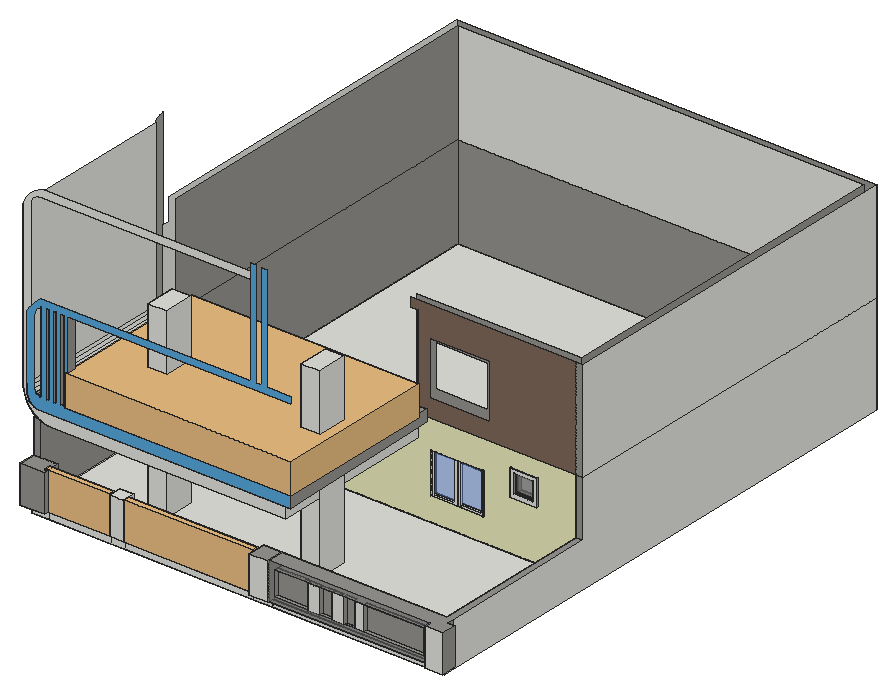
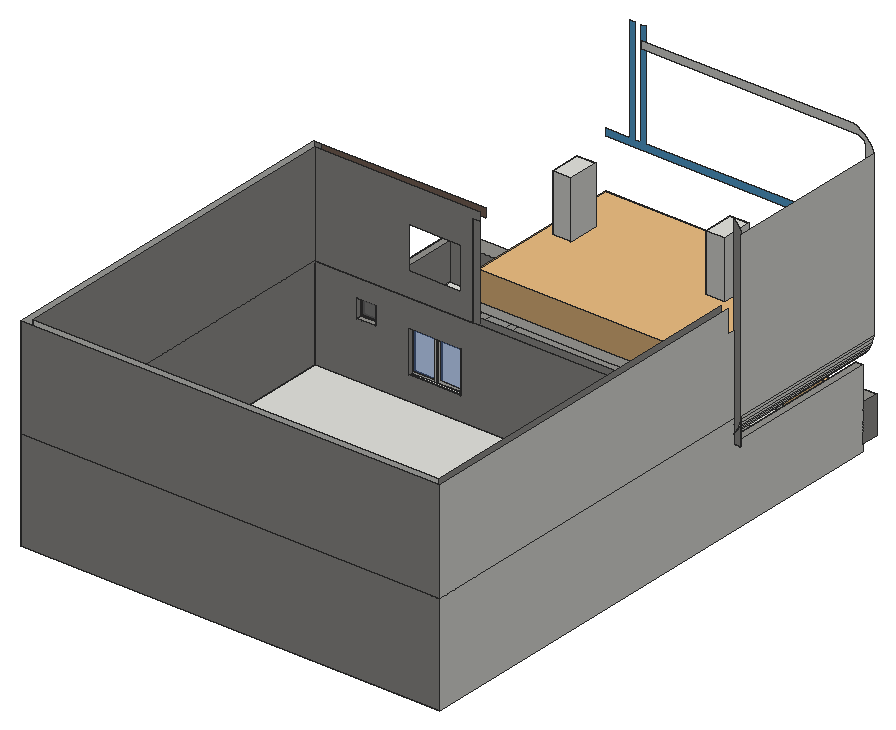
# SketchUp Ruby script. Lengths in millimetres.
U = 1.mm
M = Sketchup.active_model
def pt(a) = Geom::Point3d.new(a.map { |v| v * U })
def face(e, loops, mat)
  f = e.add_face(loops[0].map { |a| pt(a) })
  loops[1..].each { |l| e.add_face(l.map { |a| pt(a) }).erase! }
  f.material = f.back_material = mat if mat
  f
end
# faces: each face lists its corners as indices into pts; further lists are holes
def faces(e, pts, list, mat = nil) = list.each { |f| face(e, (f[0].is_a?(Array) ? f : [f]).map { |l| l.map { |i| pts[i] } }, mat) }
# xy, xz, yz: faces in a plane at the given z, y or x. An outline is a flat list of corners, or four numbers for a rectangle; further outlines are holes
def ring(l) = l.size == 4 ? [[l[0], l[1]], [l[2], l[1]], [l[2], l[3]], [l[0], l[3]]] : l.each_slice(2).to_a
def flat(e, list, mat, &to3) = list.each { |f| face(e, (f[0].is_a?(Array) ? f : [f]).map { |l| ring(l).map { |u, v| to3.(u, v) } }, mat) }
def xy(e, z, list, mat = nil) = flat(e, list, mat) { |x, y| [x, y, z] }
def xz(e, y, list, mat = nil) = flat(e, list, mat) { |x, z| [x, y, z] }
def yz(e, x, list, mat = nil) = flat(e, list, mat) { |y, z| [x, y, z] }
def lines(e, pts, list) = list.each { |a, b| e.add_line(pt(pts[a]), pt(pts[b])) }
# prism: a flat outline (further loops are holes) pulled along v
def prism(e, loops, v, mat = nil)
  f = face(e, loops, mat); d = Geom::Vector3d.new(v.map { |x| x * U })
  f.pushpull(f.normal.samedirection?(d) ? d.length : -d.length)
end
def box(e, o, s, mat = nil) = prism(e, [[o, [o[0] + s[0], o[1], o[2]], [o[0] + s[0], o[1] + s[1], o[2]], [o[0], o[1] + s[1], o[2]]]], [0, 0, s[2]], mat)
def at(x, y, z, deg = 0) = Geom::Transformation.translation(pt([x, y, z])) * Geom::Transformation.rotation(ORIGIN, Z_AXIS, deg.degrees)
def axes(o, x, y, z) = Geom::Transformation.new([*x, 0, *y, 0, *z, 0, *pt(o).to_a, 1])
def part(name) = M.definitions.add(name)
# library, detail: a bought-in or finely detailed component or shape, given as its bounding box
def library(name, o, s) = part(name).tap { |d| box(d.entities, o, s) }
def detail(e, o, s) = box(e.add_group.entities, o, s)
def put(e, d, t, mat = nil) = e.add_instance(d, t).tap { |i| i.material = mat if mat }
def group(e, t, mat = nil) = e.add_group.tap { |g| g.transformation = t; g.material = mat if mat }.entities
root = M.entities
M.materials.add("Kính").color = [128, 128, 128]
M.materials["Kính"].alpha = 0.5
M.materials.add("Nhôm singfa").color = [71, 71, 75]
M.materials.add("Polis06_194").color = [79, 50, 36]
M.materials.add("Teddy_DressDepth").color = [87, 167, 219]
M.materials.add("Teddy_Paper").color = [237, 237, 189]
M.materials.add("[Granite Brown]").color = [126, 104, 91]
M.materials.add("[Granite Light Gray]").color = [149, 148, 144]
M.materials.add("[Translucent Glass Blue]").color = [100, 149, 237]
M.materials["[Translucent Glass Blue]"].alpha = 0.5
c1 = part("Flush door")
xy(c1.entities,0,[[0,0,120,30],[0,870,120,900]],"Polis06_194")
xy(c1.entities,2165.6,[[0,30,120,870]],"Polis06_194")
xy(c1.entities,2200,[[0,0,120,900]],"Polis06_194")
xz(c1.entities,0,[[0,0,120,2200]],"Polis06_194")
xz(c1.entities,30,[[0,0,60,2165.6],[60,0,120,2165.6]],"Polis06_194")
xz(c1.entities,870,[[0,0,120,2165.6]],"Polis06_194")
xz(c1.entities,900,[[0,0,120,2200]],"Polis06_194")
yz(c1.entities,0,[[0,0,30,2200],[870,0,900,2200],[30,2165.6,870,2200]],"Polis06_194")
yz(c1.entities,60,[[30,0,870,0,870,2164.4,30,2165.6]],"Polis06_194")
yz(c1.entities,120,[[0,0,30,2200],[870,0,900,2200],[30,2165.6,870,2200]],"Polis06_194")
c2 = library("GR-Door_Half_Glass_Double_6-0x6-8",[0,0,-152.4],[2108.2,2146.3,190.5])
c3 = part("Group\#1")
box(c3.entities,[0,0,0],[617.5,999.2,6065.8])
c4 = part("Janela aluminio")
xy(c4.entities,0,[[0,0,1200,40],[600,40,1200,70],[0,70,660,100],[0,100,1200,150]])
xy(c4.entities,1100,[[0,0,1200,40],[600,40,1200,70],[0,70,0,150,1200,150,1200,100,660,100,660,70],[660,70,1200,100]])
xz(c4.entities,40,[[0,0,600,0,600,1050,540,1050,540,50,50,50,50,1050,600,1050,600,1100,0,1100],[[600,0,1200,1100],[652.8,50,1150,1050]]])
xz(c4.entities,70,[[[0,0,600,1100],[60,60,540,1040]],[600,0,660,1100]])
xz(c4.entities,70,[[60,60,540,1040]],"[Translucent Glass Blue]")
xz(c4.entities,100,[[660,0,660,60,1140,60,1140,1040,660,1040,660,1100,1200,1100,1200,0]])
xz(c4.entities,100,[[660,60,1140,1040]],"[Translucent Glass Blue]")
yz(c4.entities,0,[[0,0,40,1100],[70,0,150,1100]])
yz(c4.entities,600,[[40,0,70,1100]])
yz(c4.entities,660,[[70,0,100,1100]])
yz(c4.entities,1200,[[0,0,40,1100],[40,0,70,1100],[100,0,150,1100]])
c5 = part("Window jamb")
xz(c5.entities,0,[[0,7.1,55,62.1,55,1417.9,0,1472.9]],"Nhôm singfa")
xz(c5.entities,65,[[0,7.1,0,1472.9,55,1417.9,55,62.1]],"Nhôm singfa")
yz(c5.entities,0,[[5,0,0,7.1,0,1472.9,5,1480,60,1480,65,1472.9,65,7.1,60,0]],"Nhôm singfa")
yz(c5.entities,60,[[5,60,60,1420]],"Nhôm singfa")
p = [[55,0,62.1],[0,0,7.1],[0,5,0],[60,5,60],[60,60,60],[0,60,0],
  [0,65,7.1],[55,65,62.1],[55,0,1417.9],[60,5,1420],[55,65,1417.9],[60,60,1420],
  [0,0,1472.9],[0,5,1480],[0,65,1472.9],[0,60,1480]]
faces(c5.entities,p,[[0,1,2,3],[4,3,2,5],[6,7,4,5],[8,0,3,9],[7,10,11,4],[12,8,9,13],[10,14,15,11],[15,13,9,11]],"Nhôm singfa")
c6 = part("Window frame rail")
xy(c6.entities,0,[[7.1,0,0,5,0,60,7.1,65,1832.9,65,1840,60,1840,5,1832.9,0]],"Nhôm singfa")
xy(c6.entities,60,[[60,5,1780,60]],"Nhôm singfa")
xz(c6.entities,0,[[7.1,0,1832.9,0,1777.9,55,62.1,55]],"Nhôm singfa")
xz(c6.entities,65,[[7.1,0,62.1,55,1777.9,55,1832.9,0]],"Nhôm singfa")
p = [[7.1,0,0],[62.1,0,55],[60,5,60],[0,5,0],[1777.9,0,55],[1832.9,0,0],
  [1840,5,0],[1780,5,60],[60,60,60],[0,60,0],[1840,60,0],[1780,60,60],
  [62.1,65,55],[7.1,65,0],[1832.9,65,0],[1777.9,65,55]]
faces(c6.entities,p,[[0,1,2,3],[4,5,6,7],[2,8,9,3],[6,10,11,7],[9,8,12,13],[11,10,14,15],[1,4,7,2],[8,11,15,12]],"Nhôm singfa")
c7 = part("Vertical glazing bead")
box(c7.entities,[0,0,0],[15,10,1360],"Nhôm singfa")
c8 = part("Horizontal glazing bead")
box(c8.entities,[-1306.7,0,0],[1690,10,15],"Nhôm singfa")
c9 = part("Vertical glazing bead \#1")
box(c9.entities,[0,0,0],[15,10,1360],"Nhôm singfa")
c10 = part("Horizontal glazing bead \#1")
box(c10.entities,[-1306.7,0,0],[1690,10,15],"Nhôm singfa")
c11 = part("Glazing bead frame")
put(c11.entities,c7,axes([413.3,0,0],[-1,0,0],[0,1,0],[0,0,1]))
put(c11.entities,c8,at(15,0,1345))
put(c11.entities,c9,at(-1306.7,0,0))
put(c11.entities,c10,at(15,0,0))
c12 = part("Vertical glazing bead \#2")
box(c12.entities,[0,0,0],[15,10,1360],"Nhôm singfa")
c13 = part("Horizontal glazing bead \#2")
box(c13.entities,[-1306.7,0,0],[1690,10,15],"Nhôm singfa")
c14 = part("Vertical glazing bead \#3")
box(c14.entities,[0,0,0],[15,10,1360],"Nhôm singfa")
c15 = part("Horizontal glazing bead \#3")
box(c15.entities,[-1306.7,0,0],[1690,10,15],"Nhôm singfa")
c16 = part("Glazing bead frame \#1")
put(c16.entities,c12,axes([413.3,0,0],[-1,0,0],[0,1,0],[0,0,1]))
put(c16.entities,c13,at(15,0,1345))
put(c16.entities,c14,at(-1306.7,0,0))
put(c16.entities,c15,at(15,0,0))
c17 = part("Window pane")
box(c17.entities,[-1306.7,0,0],[1720,10,1360],"Kính")
c18 = part("Window glazing assembly")
put(c18.entities,c11,axes([0,15,0],[1,0,0],[0,-1,0],[0,0,1]))
put(c18.entities,c16,at(0,25,0))
put(c18.entities,c17,at(0,15,0))
c19 = part("Fixed window")
put(c19.entities,c5,axes([1840,0,0],[-1,0,0],[0,1,0],[0,0,1]))
put(c19.entities,c5,at(0,0,0))
put(c19.entities,c6,at(0,0,0))
put(c19.entities,c6,axes([0,0,1480],[1,0,0],[0,1,0],[0,0,-1]))
put(c19.entities,c18,at(1366.7,10,60))
c20 = part("Untitled")
put(c20.entities,c19,at(0,0,0))
c21 = library("Group\#3",[0,0,0],[7410.7,5205.1,1015.2])
xy(root,-228.6,[[482.6,355.6,482.6,6015,3911.6,6015,3911.6,6243.6,482.6,6243.6,482.6,17800.6,13766.8,17800.6,13766.8,6243.6,4826,6243.6,4826,6015,13766.8,6015,13766.8,731.8,13995.4,731.8,13995.4,355.6]])
xy(root,-228.6,[[254,731.8,254,18029.2,13995.4,18029.2,13995.4,731.8,13766.8,731.8,13766.8,17800.6,482.6,17800.6,482.6,731.8]],"[Granite Light Gray]")
xy(root,0,[[254,171.5,482.6,731.8],[3060.9,312.7,3535.5,355.6],[1041.4,355.6,3060.9,355.6,3060.9,731.8,3535.5,731.8,3535.5,355.6,7767.8,355.6,7767.8,731.8,13766.8,731.8,13766.8,6015,4826,6015,4826,6243.6,13766.8,6243.6,13766.8,17800.6,482.6,17800.6,482.6,6243.6,3911.6,6243.6,3911.6,6015,482.6,6015,482.6,731.8,1041.4,731.8],[482.6,355.6,1041.4,731.8],[3060.9,355.6,3535.5,731.8]])
xy(root,0,[[13649.6,0,13766.8,355.6],[13766.8,0,13995.4,355.6],[13995.4,0,14222.2,496.9],[7767.8,150.8,8369.5,355.6],[482.6,171.5,1041.4,355.6],
  [8369.5,198.4,13649.6,355.6],[7767.8,355.6,8369.5,731.8],[8369.5,355.6,13995.4,731.8],[482.6,6015,3911.6,6243.6],[4826,6015,13766.8,6243.6]],"[Granite Light Gray]")
xy(root,204.6,[[9655,171.5,10050.7,198.4],[10431.7,182.6,10847.2,198.4],[8574.1,198.4,9655,312.7],[9655,198.4,10050.7,198.4,10050.7,312.7,10431.7,312.7,10431.7,198.4,10847.2,198.4,10847.2,312.7,11170.1,312.7,11170.1,198.4,11490.1,198.4,11490.1,312.7,13444.9,312.7,13444.9,496.9,8574.1,496.9,8574.1,312.7,9655,312.7],[10050.7,198.4,10431.7,312.7],
  [10847.2,198.4,11170.1,312.7],[11490.1,198.4,13444.9,312.7]],"[Granite Light Gray]")
xy(root,757.2,[[9005,6015,10719.5,6243.6]],"[Granite Light Gray]")
xy(root,914.4,[[982.8,6015,1897.2,6243.6]],"[Granite Light Gray]")
xy(root,1014.6,[[9655,171.5,9918.6,198.4],[9918.6,171.5,10050.7,198.4],[10431.7,182.6,10717.5,198.4],[10717.5,182.6,10847.2,198.4],[10717.5,198.4,10717.5,312.7,8574.1,312.7,8574.1,496.9,13444.9,496.9,13444.9,312.7,11490.1,312.7,11490.1,198.4,11170.1,198.4,11170.1,312.7,10847.2,312.7,10847.2,198.4],
  [8574.1,198.4,9543.8,312.7],[9543.8,198.4,9655,312.7],[9655,198.4,9918.6,312.7],[9918.6,198.4,10050.7,312.7],[10050.7,198.4,10337.7,312.7],
  [10337.7,198.4,10431.7,312.7],[10431.7,198.4,10717.5,312.7],[10847.2,198.4,11170.1,312.7],[11490.1,198.4,13444.9,312.7]],"[Granite Light Gray]")
xy(root,1219.2,[[3060.9,312.7,3535.5,731.8]])
xy(root,1219.2,[[13649.6,0,14222.2,0,14222.2,496.9,13995.4,496.9,13995.4,6015,13766.8,6015,13766.8,731.8,8369.5,731.8,8369.5,198.4,13649.6,198.4],[7767.8,150.8,8369.5,731.8],[254,171.5,1041.4,731.8]],"[Granite Light Gray]")
xy(root,1692.4,[[11641.3,5957.9,12530.3,6015]],"[Granite Light Gray]")
xy(root,1827.3,[[11797.2,5957.9,12406.8,6243.6]],"[Granite Light Gray]")
xy(root,2133.6,[[982.8,6015,1897.2,6243.6],[3911.6,6015,4826,6243.6],[9005,6015,10719.5,6243.6]],"[Granite Light Gray]")
xy(root,2324.9,[[822.8,604.8,8363.8,6014.8],[8363.8,604.8,8592.4,6015],[254,731.8,482.6,6014.8],[0,6014.8,254,6015],[254,6014.8,482.6,6015],
  [482.6,6014.8,8363.8,6015]],"[Granite Light Gray]")
xy(root,2438.4,[[11797.2,5957.9,12406.8,6243.6]],"[Granite Light Gray]")
xy(root,2533.7,[[11641.3,5957.9,12530.3,6015]],"[Granite Light Gray]")
xy(root,2806.5,[[629.1,442.9,629.1,604.8,8592.4,604.8,8592.4,731.8,8897.2,731.8,8897.2,442.9]],"[Granite Light Gray]")
xy(root,2895.6,[[881.7,6014.8,8363.8,6015]],"[Granite Light Gray]")
xy(root,3048,[[254,6015,254,18029.2,13995.4,18029.2,13995.4,6015,13766.8,6015,13766.8,17800.6,482.6,17800.6,482.6,6015],[482.6,6015,4826,6243.6],[4826,6015,8363.8,6243.6],[8363.8,6015,8592.4,6243.6],[8592.4,6015,13766.8,6243.6]],"[Granite Light Gray]")
xy(root,3200.4,[[905.1,442.9,961.7,731.8],[1150.1,442.9,1205.9,731.8],[1348.7,442.9,1445.7,731.8],[1577.5,442.9,8897.2,731.8],[482.6,731.8,716.7,6014.8]],"[Granite Light Gray]")
xz(root,0,[[13649.6,0,14222.2,1219.2]])
xz(root,150.8,[[7767.8,0,8369.5,1219.2]])
xz(root,171.5,[[9655,204.6,10050.7,1014.6]])
xz(root,171.5,[[254,0,1041.4,1219.2]],"[Granite Light Gray]")
xz(root,182.6,[[10431.7,204.6,10847.2,1014.6]])
xz(root,198.4,[[11170.1,204.6,11490.1,1014.6]])
xz(root,198.4,[[[8369.5,0,13649.6,1219.2],[8574.1,204.6,13444.9,1014.6]]],"Kính")
xz(root,312.7,[[3060.9,0,3535.5,1219.2]])
xz(root,312.7,[[8574.1,204.6,9655,1014.6],[10050.7,204.6,10431.7,1014.6],[10847.2,204.6,11170.1,1014.6],[11490.1,204.6,13444.9,1014.6]],"[Granite Light Gray]")
xz(root,355.6,[[482.6,-228.6,1041.4,0],[1041.4,-228.6,3060.9,0],[3060.9,-228.6,3535.5,0],[3535.5,-228.6,7767.8,0],[7767.8,-228.6,8369.5,0],
  [8369.5,-228.6,13995.4,0]])
xz(root,442.9,[[[629.1,2806.5,8897.2,2806.5,8897.2,3200.4,1577.5,3200.4,1577.5,5867.4,8897.2,5867.4,8897.2,6096,8096.7,6096,8096.7,9540.9,7934.7,9540.9,7934.7,6096,7749.9,6096,7749.9,9540.9,7588,9540.9,7588,6096,718.4,6096,677,6055.4,636.1,6014.4,595.7,5972.9,555.7,5930.9,516.3,5888.5,477.3,5845.6,438.8,5802.3,400.8,5758.5,363.3,5714.3,326.4,5669.7,289.9,5624.7,254,5579.2,254,3201.2,257.2,3151.2,266.6,3102.1,282.2,3054.6,303.6,3009.4,330.6,2967.3,362.7,2928.9,399.4,2894.9,440.1,2865.8,484.2,2842.1,530.8,2824.1,579.4,2812.2],[716.7,3200.4,686.1,3202.4,656.1,3208.4,627.1,3218.3,599.6,3231.8,574.2,3248.8,551.2,3269,531,3292,514,3317.5,500.4,3344.9,490.6,3373.9,484.6,3404,482.6,3434.5,482.6,5493.5,485.8,5542.3,495.3,5590.3,511.1,5636.6,532.7,5680.5,559.9,5721.1,592.1,5757.9,628.9,5790.1,669.5,5817.3,713.4,5838.9,716.7,5840.1,759.7,5854.7,807.7,5864.2,856.5,5867.4,961.7,5867.4,961.7,3200.4,905.1,3200.4,905.1,5840.1,716.7,5840.1],[1348.7,3200.4,1445.7,5867.4],[1150.1,3200.4,1205.9,5867.4]]],"Teddy_DressDepth")
xz(root,496.9,[[13995.4,0,14222.2,1219.2],[8574.1,204.6,13444.9,1014.6]],"[Granite Light Gray]")
xz(root,604.8,[[822.8,2324.9,8592.4,2324.9,8592.4,2806.5,629.1,2806.5,579.4,2812.2,530.8,2824.1,484.2,2842.1,440.1,2865.8,399.4,2894.9,362.7,2928.9,330.6,2967.3,303.6,3009.4,282.2,3054.6,266.6,3102.1,257.2,3151.2,254,3201.2,254,8655.7,256.5,8693.6,263.9,8730.9,276.1,8766.9,292.9,8801,314.1,8832.6,339.1,8861.2,367.7,8886.3,399.3,8907.4,433.4,8924.2,469.4,8936.4,506.7,8943.8,544.6,8946.3,7588,8946.3,7588,9200.3,665.2,9200.3,589.2,9171.7,515.6,9137.3,444.8,9097.3,377.4,9051.9,313.6,9001.5,254,8946.3,198.8,8886.7,148.4,8822.9,103,8755.5,63,8684.8,28.6,8611.1,0,8535.1,0,3200.4,13.2,3092.8,38.6,2987.3,76,2885.5,124.9,2788.6,184.5,2698,254.1,2614.8,332.8,2540.2,419.6,2475,513.2,2420.3,612.5,2376.7,716.2,2344.7]])
xz(root,731.8,[[13766.8,-228.6,13995.4,0],[3060.9,0,3535.5,1219.2]])
xz(root,731.8,[[254,-228.6,482.6,0],[254,0,482.6,1219.2],[482.6,0,1041.4,1219.2],[7767.8,0,8369.5,1219.2],[8369.5,0,13766.8,1219.2],
  [254,1219.2,482.6,2324.9],[716.7,3200.4,905.1,5840.1],[961.7,3200.4,1150.1,5867.4],[1205.9,3200.4,1348.7,5867.4],[1445.7,3200.4,1577.5,5867.4]],"[Granite Light Gray]")
xz(root,5957.9,[[[11641.3,1692.4,12530.3,2533.7],[11797.2,1827.3,12406.8,2438.4]]])
xz(root,6014.8,[[0,2324.9,254,2324.9,254,2614.9,184.5,2698,124.9,2788.6,76,2885.5,38.6,2987.3,13.2,3092.8,0,3200.4],[254,2324.9,822.8,2324.9,716.2,2344.7,612.5,2376.7,513.2,2420.3,419.6,2475,332.8,2540.2,254.1,2614.8,254,2614.9],[822.8,2324.9,8363.8,2324.9,8363.8,2895.6,254,2895.6,254,2614.9,254.1,2614.8,332.8,2540.2,419.6,2475,513.2,2420.3,612.5,2376.7,716.2,2344.7],[254,2895.6,881.7,2895.6,806.9,2900,733.1,2913.2,661.5,2935,592.8,2965.1,528.2,3003,468.5,3048.3,414.6,3100.3,367.2,3158.2,326.9,3221.4,294.3,3288.9,269.9,3359.7,254,3432.9],[482.6,3200.4,482.6,3341.1,551.2,3269,574.2,3248.8,599.6,3231.8,627.1,3218.3,656.1,3208.4,686.1,3202.4,716.7,3200.4]],"[Granite Light Gray]")
xz(root,6015,[[482.6,-228.6,3911.6,0],[4826,-228.6,13766.8,0]])
xz(root,6015,[[[4826,0,13766.8,0,13766.8,3048,8897.2,3048,8897.2,2907.4,8592.4,2907.4,8592.4,2324.9,8363.8,2324.9,8363.8,2172.5,4826,2172.5],[9005,757.2,10719.5,2133.6],[11641.3,1692.4,12530.3,2533.7]]],"Teddy_Paper")
xz(root,6015,[[[8592.4,3048,13766.8,3048,13766.8,6378.2,8363.8,6378.2,8363.8,6096,8592.4,6096],[8973.7,3629.7,10939,5406.1]]],"[Granite Brown]")
xz(root,6015,[[482.6,0,3911.6,0,3911.6,2172.5,1897.2,2172.5,1897.2,914.4,982.8,914.4,982.8,2172.5,8363.8,2172.5,8363.8,2324.9,482.6,2324.9],[13766.8,1219.2,13995.4,3048],[982.8,2133.6,1897.2,2172.5],[3911.6,2133.6,4826,2172.5],[0,2324.9,0,8535.1,28.6,8611.1,63,8684.8,103,8755.5,148.4,8822.9,198.8,8886.7,254,8946.3,254,2324.9],
  [254,2324.9,482.6,2895.6],[482.6,2324.9,8363.8,2895.6],[8363.8,2324.9,8592.4,2324.9,8592.4,2907.4,8897.2,2907.4,8897.2,3048,8363.8,3048],[254,2895.6,482.6,2895.6,482.6,3037.6,468.9,3048,254,3048],[482.6,2895.6,881.7,2895.6,806.9,2900,733.1,2913.2,661.5,2935,592.8,2965.1,528.2,3003,482.6,3037.6],
  [881.7,2895.6,4826,2895.6,4826,3048,482.6,3048,482.6,3037.6,528.2,3003,592.8,2965.1,661.5,2935,733.1,2913.2,806.9,2900],[4826,2895.6,8363.8,3048],[482.6,3037.6,482.6,3048,468.9,3048],[254,3048,468.9,3048,468.5,3048.3,414.6,3100.3,367.2,3158.2,326.9,3221.4,294.3,3288.9,269.9,3359.7,254,3432.9],[13766.8,3048,13995.4,6378.2]],"[Granite Light Gray]")
xz(root,6243.6,[[482.6,-228.6,3911.6,0],[4826,-228.6,13766.8,0]])
xz(root,6243.6,[[[482.6,0,482.6,3048,13766.8,3048,13766.8,0,4826,0,4826,2133.6,3911.6,2133.6,3911.6,0],[9005,757.2,10719.5,2133.6],[982.8,914.4,1897.2,2133.6],[11797.2,1827.3,12406.8,2438.4]],[482.6,3048,8363.8,3276.6],[8363.8,3048,8592.4,6096],[[8592.4,3048,8592.4,6096,8363.8,6096,8363.8,6378.2,13766.8,6378.2,13766.8,3048],[9005,3805.2,10719.5,5181.6]]],"[Granite Light Gray]")
xz(root,17800.6,[[482.6,-228.6,13766.8,0],[482.6,3048,13766.8,6378.2]])
xz(root,17800.6,[[482.6,0,13766.8,3048]],"[Granite Light Gray]")
xz(root,18029.2,[[254,-228.6,13995.4,3048],[254,3048,13995.4,6378.2]],"[Granite Light Gray]")
yz(root,0,[[6014.8,2324.9,6014.8,3200.4,604.8,3200.4,604.8,8535.1,6015,8535.1,6015,2324.9]])
yz(root,254,[[731.8,-228.6,731.8,2324.9,6015,2324.9,6015,3048,18029.2,3048,18029.2,-228.6],[6015,3048,6015,5631.6,6243.6,5631.6,6243.6,6378.2,18029.2,6378.2,18029.2,3048]])
yz(root,254,[[171.5,0,731.8,1219.2],[6014.8,2324.9,6015,3432.9],[442.9,3201.2,604.8,3432.9]],"[Granite Light Gray]")
yz(root,482.6,[[355.6,-228.6,731.8,0],[731.8,-228.6,6015,0],[6243.6,-228.6,17800.6,0]])
yz(root,482.6,[[6015,-228.6,6243.6,0],[731.8,0,6015,2324.9],[6015,0,6243.6,3048],[6243.6,0,17800.6,3048],[6243.6,3048,17800.6,6378.2],
  [731.8,3200.4,6014.8,3276.6,6014.8,3200.4]],"[Granite Light Gray]")
yz(root,716.7,[[442.9,3200.4,731.8,5840.1]],"[Granite Light Gray]")
yz(root,905.1,[[442.9,3200.4,731.8,5840.1]],"[Granite Light Gray]")
yz(root,910.5,[[5405.4,2171.4,6015,2172.5,6014.8,2324.9,5405.2,2323.8]],"[Granite Light Gray]")
yz(root,961.7,[[442.9,3200.4,731.8,5867.4]],"[Granite Light Gray]")
yz(root,982.8,[[6015,914.4,6243.6,2133.6]],"[Granite Light Gray]")
yz(root,1041.4,[[171.5,0,731.8,1219.2]],"[Granite Light Gray]")
yz(root,1150.1,[[442.9,3200.4,731.8,5867.4]],"[Granite Light Gray]")
yz(root,1205.9,[[442.9,3200.4,731.8,5867.4]],"[Granite Light Gray]")
yz(root,1348.7,[[442.9,3200.4,731.8,5867.4]],"[Granite Light Gray]")
yz(root,1445.7,[[442.9,3200.4,731.8,5867.4]],"[Granite Light Gray]")
yz(root,1577.5,[[442.9,3200.4,731.8,5867.4]],"[Granite Light Gray]")
yz(root,1897.2,[[6015,914.4,6243.6,2133.6]],"[Granite Light Gray]")
yz(root,3060.9,[[312.7,0,731.8,1219.2]])
yz(root,3535.5,[[312.7,0,731.8,1219.2]])
yz(root,3911.6,[[6015,-228.6,6243.6,0]])
yz(root,3911.6,[[6015,0,6243.6,2133.6]],"[Granite Light Gray]")
yz(root,4826,[[6015,-228.6,6243.6,0]])
yz(root,4826,[[6015,0,6243.6,2133.6]],"[Granite Light Gray]")
yz(root,7767.8,[[150.8,0,731.8,1219.2]],"[Granite Light Gray]")
yz(root,8363.8,[[5405.4,2171.4,5405.2,2323.8,6014.8,2324.9,6015,2324.9,6015,2172.5],[6014.8,2324.9,6015,2895.6]],"[Granite Light Gray]")
yz(root,8369.5,[[150.8,0,198.4,1219.2],[198.4,0,731.8,1219.2]],"[Granite Light Gray]")
yz(root,8574.1,[[198.4,204.6,312.7,1014.6],[312.7,204.6,496.9,1014.6]],"[Granite Light Gray]")
yz(root,8592.4,[[604.8,2324.9,6015,2324.9,6015,2907.4,731.8,2806.5,604.8,2806.5]])
yz(root,8592.4,[[6015,3048,6015,6096,6013,6096,6013.2,5867.4,6014.9,3276.6],[6015,3048,6243.6,6096]],"[Granite Light Gray]")
yz(root,8897.2,[[442.9,2806.5,731.8,2806.5,6015,2907.4,6015,3048,6014.9,3276.6,731.8,3200.4,442.9,3200.4]],"[Granite Light Gray]")
yz(root,9005,[[6015,757.2,6243.6,2133.6]],"[Granite Light Gray]")
yz(root,9655,[[171.5,204.6,312.7,1014.6]],"[Granite Light Gray]")
yz(root,10050.7,[[171.5,204.6,312.7,1014.6]],"[Granite Light Gray]")
yz(root,10431.7,[[182.6,204.6,312.7,1014.6]],"[Granite Light Gray]")
yz(root,10719.5,[[6015,757.2,6243.6,2133.6]],"[Granite Light Gray]")
yz(root,10847.2,[[182.6,204.6,312.7,1014.6]],"[Granite Light Gray]")
yz(root,11170.1,[[198.4,204.6,312.7,1014.6]],"[Granite Light Gray]")
yz(root,11490.1,[[198.4,204.6,312.7,1014.6]],"[Granite Light Gray]")
yz(root,11641.3,[[5957.9,1692.4,6015,2533.7]],"[Granite Light Gray]")
yz(root,11797.2,[[5957.9,1827.3,6243.6,2438.4]],"[Granite Light Gray]")
yz(root,12406.8,[[5957.9,1827.3,6243.6,1828.8],[5957.9,1828.8,6243.6,2438.4]],"[Granite Light Gray]")
yz(root,12530.3,[[5957.9,1692.4,6015,2533.7]],"[Granite Light Gray]")
yz(root,13444.9,[[198.4,204.6,312.7,1014.6],[312.7,204.6,496.9,1014.6]],"[Granite Light Gray]")
yz(root,13649.6,[[0,0,198.4,1219.2]],"[Granite Light Gray]")
yz(root,13766.8,[[731.8,-228.6,6015,0],[6243.6,-228.6,17800.6,0]])
yz(root,13766.8,[[6015,-228.6,6243.6,0],[731.8,0,6015,1219.2],[6015,0,6243.6,3048],[6243.6,0,17800.6,3048],[6243.6,3048,17800.6,6378.2]],"[Granite Light Gray]")
yz(root,13995.4,[[355.6,-228.6,731.8,0],[731.8,-228.6,18029.2,-228.6,18029.2,3048,6015,3048,6015,1219.2,731.8,1219.2],[6015,3048,18029.2,6378.2]])
yz(root,13995.4,[[496.9,0,731.8,1219.2]],"[Granite Light Gray]")
yz(root,14222.2,[[0,0,496.9,1219.2]],"[Granite Light Gray]")
p = [[9918.6,496.9,204.6],[9918.6,312.7,1014.6],[9655,312.7,1014.6],[9543.8,312.7,1014.6],[9543.8,496.9,204.6],[10337.7,496.9,204.6],
  [10337.7,312.7,1014.6],[10050.7,312.7,1014.6],[10717.5,496.9,204.6],[10717.5,312.7,1014.6],[10431.7,312.7,1014.6],[8363.8,5405.2,2323.8],
  [8363.8,5405.4,2171.4],[4826,5405.4,2171.4],[3911.6,5405.4,2171.4],[1897.2,5405.4,2171.4],[982.8,5405.4,2171.4],[910.5,5405.4,2171.4],
  [910.5,5405.2,2323.8],[982.8,6015,2172.5],[910.5,6015,2172.5],[1897.2,6015,2172.5],[3911.6,6015,2172.5],[4826,6015,2172.5],
  [8363.8,6015,2172.5],[910.5,6014.8,2324.9],[8363.8,6014.8,2324.9],[822.8,6014.8,2324.9],[822.8,604.8,2324.9],[716.2,604.8,2344.7],
  [716.2,6014.8,2344.7],[612.5,604.8,2376.7],[612.5,6014.8,2376.7],[513.2,604.8,2420.3],[513.2,6014.8,2420.3],[419.6,604.8,2475],
  [419.6,6014.8,2475],[332.8,604.8,2540.2],[332.8,6014.8,2540.2],[254.1,604.8,2614.8],[254.1,6014.8,2614.8],[184.5,604.8,2698],
  [184.5,6014.8,2698],[254,6014.8,2614.9],[124.9,604.8,2788.6],[124.9,6014.8,2788.6],[76,604.8,2885.5],[76,6014.8,2885.5],
  [579.4,442.9,2812.2],[579.4,604.8,2812.2],[629.1,604.8,2806.5],[629.1,442.9,2806.5],[8592.4,731.8,2806.5],[8592.4,6015,2907.4],
  [8897.2,6015,2907.4],[8897.2,731.8,2806.5],[530.8,442.9,2824.1],[530.8,604.8,2824.1],[484.2,442.9,2842.1],[484.2,604.8,2842.1],
  [440.1,442.9,2865.8],[440.1,604.8,2865.8],[399.4,442.9,2894.9],[399.4,604.8,2894.9],[38.6,604.8,2987.3],[38.6,6014.8,2987.3],
  [362.7,442.9,2928.9],[362.7,604.8,2928.9],[881.7,6015,2895.6],[881.7,6014.8,2895.6],[806.9,6014.8,2900],[806.9,6015,2900],
  [770,6014.8,2906.6],[733.1,6014.8,2913.2],[733.1,6015,2913.2],[661.5,6014.8,2935],[661.5,6015,2935],[330.6,442.9,2967.3],
  [330.6,604.8,2967.3],[592.8,6014.8,2965.1],[592.8,6015,2965.1],[528.2,6014.8,3003],[528.2,6015,3003],[303.6,442.9,3009.4],
  [303.6,604.8,3009.4],[13.2,604.8,3092.8],[13.2,6014.8,3092.8],[468.5,6014.8,3048.3],[468.5,6015,3048.3],[468.9,6015,3048],
  [482.6,6015,3037.6],[282.2,442.9,3054.6],[282.2,604.8,3054.6],[8592.4,6015,3048],[8592.4,6014.9,3276.6],[8897.2,6014.9,3276.6],
  [8897.2,6015,3048],[414.6,6014.8,3100.3],[414.6,6015,3100.3],[266.6,442.9,3102.1],[266.6,604.8,3102.1],[0,604.8,3200.4],
  [0,6014.8,3200.4],[367.2,6014.8,3158.2],[367.2,6015,3158.2],[257.2,442.9,3151.2],[257.2,604.8,3151.2],[254,442.9,3201.2],
  [254,604.8,3201.2],[326.9,6014.8,3221.4],[326.9,6015,3221.4],[686.1,6014.8,3202.4],[686.1,442.9,3202.4],[716.7,442.9,3200.4],
  [716.7,731.8,3200.4],[716.7,6014.8,3200.4],[482.6,6014.9,3276.6],[482.6,6014.8,3276.6],[482.6,731.8,3200.4],[905.1,731.8,3200.4],
  [961.7,731.8,3200.4],[1150.1,731.8,3200.4],[1205.9,731.8,3200.4],[1348.7,731.8,3200.4],[1445.7,731.8,3200.4],[1577.5,731.8,3200.4],
  [8897.2,731.8,3200.4],[4237,6014.9,3276.6],[3170.2,6014.9,3276.6],[656.1,6014.8,3208.4],[656.1,442.9,3208.4],[627.1,6014.8,3218.3],
  [627.1,442.9,3218.3],[599.6,6014.8,3231.8],[599.6,442.9,3231.8],[294.3,6014.8,3288.9],[294.3,6015,3288.9],[574.2,6014.8,3248.8],
  [574.2,442.9,3248.8],[551.2,6014.8,3269],[551.2,442.9,3269],[770,731.8,2906.6],[254,731.8,2895.6],[254,6014.8,2895.6]]
faces(root,p,[[0,1,2,3,4],[5,6,7,1,0],[6,5,8,9,10],[11,12,13,14,15,16,17,18],[19,20,17,16],[21,19,16,15],[22,21,15,14],[23,22,14,13],
  [24,23,13,12],[25,26,11,18],[48,49,50,51],[52,53,54,55],[56,57,49,48],[58,59,57,56],[60,61,59,58],[62,63,61,60],
  [66,67,63,62],[68,69,70,71],[70,72,73,74,71],[74,73,75,76],[77,78,67,66],[76,75,79,80],[80,79,81,82],[83,84,78,77],
  [82,81,87,88,89,90],[91,92,84,83],[93,94,95,96],[88,87,97,98],[99,100,92,91],[98,97,103,104],[105,106,100,99],[107,108,106,105],
  [104,103,109,110],[111,112,113,114,115],[116,117,118,114,119,120,121,122,123,124,125,126,95,94,127,128],[129,130,112,111],[131,132,130,129],[133,134,132,131],[110,109,135,136],[137,138,134,133],
  [139,140,138,137]],"[Granite Light Gray]")
faces(root,p,[[27,28,29,30],[30,29,31,32],[32,31,33,34],[34,33,35,36],[36,35,37,38],[38,37,39,40],[40,39,41,42,43],[42,41,44,45],
  [45,44,46,47],[47,46,64,65],[65,64,85,86],[86,85,101,102]])
lines(root,p,[[141,72],[142,143]])
put(root,c1,axes([4826,6015,0],[0,1,0],[-1,0,0],[0,0,0.96982]))
put(root,c2,axes([952.7,350.8,0],[1,0,0],[0,0,0.578],[0,-1,0]))
put(root,c2,axes([3535.5,350.8,0],[2,0,0],[0,0,0.578],[0,-1,0]))
put(root,c3,at(2973.2,1989.8,0))
put(root,c3,at(7987.7,1989.8,0))
put(root,c4,axes([9005,6015,757.2],[1.45,0,0],[0,1,0],[0,0,1.25124]))
put(root,c4,axes([982.8,6015,914.4],[0.762,0,0],[0,1,0],[0,0,1.14372]))
put(root,c20,axes([11797.2,6015,1827.3],[0.3313,0,0],[0,1,0],[0,0,0.41294]))
put(root,c21,at(1526.5,402.9,3200.4))
